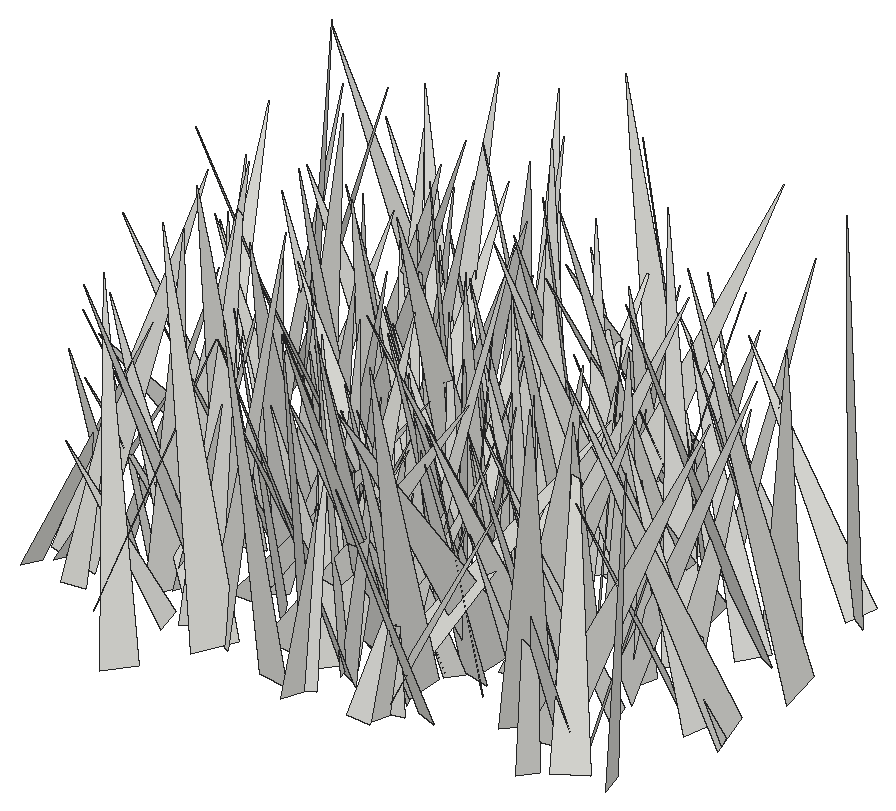
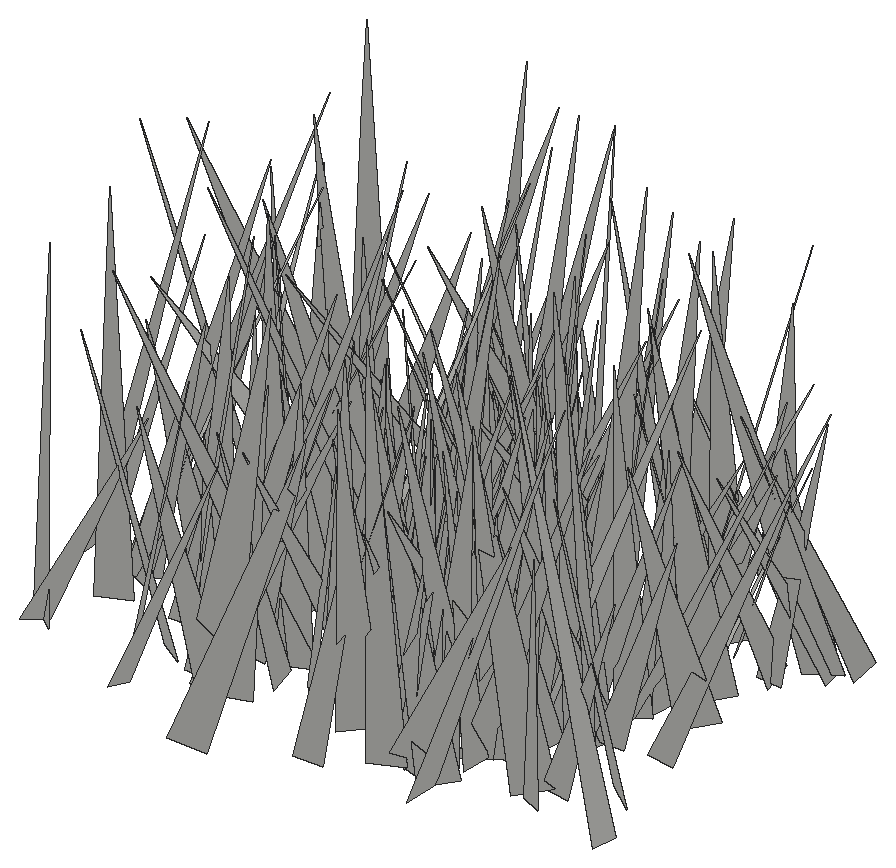
# SketchUp Ruby script. Lengths in inches.
U = 1.inch
M = Sketchup.active_model
def pt(a) = Geom::Point3d.new(a.map { |v| v * U })
def face(e, loops, mat)
  f = e.add_face(loops[0].map { |a| pt(a) })
  loops[1..].each { |l| e.add_face(l.map { |a| pt(a) }).erase! }
  f.material = f.back_material = mat if mat
  f
end
# faces: each face lists its corners as indices into pts; further lists are holes
def faces(e, pts, list, mat = nil) = list.each { |f| face(e, (f[0].is_a?(Array) ? f : [f]).map { |l| l.map { |i| pts[i] } }, mat) }
# xy, xz, yz: faces in a plane at the given z, y or x. An outline is a flat list of corners, or four numbers for a rectangle; further outlines are holes
def ring(l) = l.size == 4 ? [[l[0], l[1]], [l[2], l[1]], [l[2], l[3]], [l[0], l[3]]] : l.each_slice(2).to_a
def flat(e, list, mat, &to3) = list.each { |f| face(e, (f[0].is_a?(Array) ? f : [f]).map { |l| ring(l).map { |u, v| to3.(u, v) } }, mat) }
def xy(e, z, list, mat = nil) = flat(e, list, mat) { |x, y| [x, y, z] }
def xz(e, y, list, mat = nil) = flat(e, list, mat) { |x, z| [x, y, z] }
def yz(e, x, list, mat = nil) = flat(e, list, mat) { |y, z| [x, y, z] }
def lines(e, pts, list) = list.each { |a, b| e.add_line(pt(pts[a]), pt(pts[b])) }
# prism: a flat outline (further loops are holes) pulled along v
def prism(e, loops, v, mat = nil)
  f = face(e, loops, mat); d = Geom::Vector3d.new(v.map { |x| x * U })
  f.pushpull(f.normal.samedirection?(d) ? d.length : -d.length)
end
def box(e, o, s, mat = nil) = prism(e, [[o, [o[0] + s[0], o[1], o[2]], [o[0] + s[0], o[1] + s[1], o[2]], [o[0], o[1] + s[1], o[2]]]], [0, 0, s[2]], mat)
def at(x, y, z, deg = 0) = Geom::Transformation.translation(pt([x, y, z])) * Geom::Transformation.rotation(ORIGIN, Z_AXIS, deg.degrees)
def axes(o, x, y, z) = Geom::Transformation.new([*x, 0, *y, 0, *z, 0, *pt(o).to_a, 1])
def part(name) = M.definitions.add(name)
# library, detail: a bought-in or finely detailed component or shape, given as its bounding box
def library(name, o, s) = part(name).tap { |d| box(d.entities, o, s) }
def detail(e, o, s) = box(e.add_group.entities, o, s)
def put(e, d, t, mat = nil) = e.add_instance(d, t).tap { |i| i.material = mat if mat }
def group(e, t, mat = nil) = e.add_group.tap { |g| g.transformation = t; g.material = mat if mat }.entities
root = M.entities
c1 = part("fur_instance\#9")
p = [[0.8125,0,1.79],[0.67,-0.02,1.48],[0,-0.11,0],[0,0.11,0]]
faces(c1.entities,p,[[0,1,2,3]])
put(root,c1,axes([95.03,323.03,-27.1],[-6.05277,2.56522,0.71834],[2.46544,6.06973,-0.90131],[1.00895,0.55714,6.51184]))
put(root,c1,axes([100.52,325.12,-27.1],[3.76138,-1.24538,0.93866],[-1.27843,-3.86595,-0.00634],[-0.89313,0.28885,3.96218]))
put(root,c1,axes([94.32,326.4375,-27.1],[-3.93279,-0.23592,0.50656],[-0.05149,3.7386,1.34138],[0.55643,-1.32147,3.70448]))
put(root,c1,axes([99.45,325.49,-27.1],[1.25077,5.74635,3.18749],[6.40163,-1.79789,0.7292],[-1.48314,-2.91412,5.83551]))
put(root,c1,axes([99.67,326.98,-27.1],[6.5233,2.37968,3.04495],[3.30026,-6.53866,-1.96019],[-2.01069,-3.01183,6.66138]))
put(root,c1,axes([103.65,327.73,-27.1],[7.48346,-2.4752,1.75576],[-1.96533,-7.51292,-2.21472],[-2.31232,-1.62508,7.56464]))
put(root,c1,axes([104.87,326.64,-27.1],[-1.89303,-4.40404,0.51291],[-4.43222,1.86471,-0.34716],[-0.11875,0.60786,4.78107]))
put(root,c1,axes([103.4,327.9,-27.1],[-5.97447,-2.65496,2.2585],[-2.10106,6.3191,1.8704],[2.78122,-0.92951,6.26456]))
put(root,c1,axes([107.73,328.23,-27.1],[5.80631,-5.6916,0.53269],[-5.68589,-5.82856,-0.29992],[-0.59055,0.15799,8.12513]))
put(root,c1,axes([103.21,325.18,-27.1],[-0.85161,3.55792,0.87868],[3.50079,1.05663,-0.88551],[1.08413,-0.61714,3.54963]))
put(root,c1,axes([103.73,325.76,-27.1],[3.9323,-0.29865,1.47953],[-0.48436,-4.16008,0.44758],[-1.42954,0.58799,3.91814]))
put(root,c1,axes([96.6,326,-27.1],[5.34271,-3.44394,4.19103],[-3.85612,-6.54857,-0.46545],[-3.8152,1.796,6.33945]))
put(root,c1,axes([100.63,325.57,-27.1],[-2.63101,2.88231,1.12737],[2.88894,2.81797,-0.46255],[1.11028,-0.50218,3.87505]))
put(root,c1,axes([101.61,329.17,-27.1],[-1.56855,-7.63886,0.47282],[-7.63369,1.59619,0.46371],[0.55001,0.36889,7.78444]))
put(root,c1,axes([101.04,329.05,-27.1],[-1.24529,-7.71146,0.7872],[-7.61167,1.36728,1.35282],[1.46589,0.54863,7.69333]))
put(root,c1,axes([103.93,326.13,-27.1],[-0.42673,3.51272,1.26133],[3.73148,0.37463,0.21911],[-0.0791,-1.27778,3.53176]))
put(root,c1,axes([93.95,328.97,-27.1],[-5.87667,-3.9224,1.1719],[-3.54254,5.90008,1.98324],[2.05159,-1.04767,6.78139]))
put(root,c1,axes([104.39,331.31,-27.1],[6.48177,-5.01878,0.45242],[-4.24735,-5.8379,-3.90962],[-2.71162,-2.85253,7.2053]))
put(root,c1,axes([90.46,326.36,-27.1],[1.50954,-3.07856,1.78204],[-3.55315,-1.39659,0.59714],[-0.16832,1.87187,3.37633]))
put(root,c1,axes([103.32,326.4,-27.1],[4.26257,2.91433,0.00484],[2.86478,-4.18851,-0.95515],[0.53516,-0.79116,5.0745]))
put(root,c1,axes([101.18,327.18,-27.1],[-4.07281,-4.5818,0.7427],[-4.55178,3.7491,-1.83244],[-0.90871,1.75604,5.85003]))
put(root,c1,axes([110.46,327.26,-27.1],[-2.82559,-5.19892,1.36333],[-5.31081,2.46391,-1.61114],[-0.82624,1.9421,5.69358]))
put(root,c1,axes([101.12,327.32,-27.1],[-2.2184,-4.85625,2.50772],[-5.03427,2.86928,1.10295],[2.1279,1.72546,5.22379]))
put(root,c1,axes([91.81,325.9,-27.1],[4.67763,2.46387,0.32375],[2.42875,-4.67875,0.51598],[-0.52599,0.30722,5.26162]))
put(root,c1,axes([96.28,326.54,-27.1],[3.51282,6.48869,2.15536],[6.79895,-3.57131,-0.32959],[-0.72316,-2.057,7.37118]))
put(root,c1,axes([101.98,329.83,-27.1],[0.91658,-6.09487,0.23316],[-5.96683,-0.94489,-1.24341],[-1.26442,0.04079,6.03668]))
put(root,c1,axes([112.29,326.99,-27.1],[-4.83531,-1.63891,2.39644],[-2.01972,5.24312,-0.48946],[2.08559,1.27782,5.08199]))
put(root,c1,axes([93.04,327.95,-27.1],[-5.61419,2.77509,3.47904],[3.15086,6.4338,-0.04739],[3.14276,-1.49299,6.26243]))
put(root,c1,axes([94.93,328.77,-27.1],[-3.76268,-4.24685,0.11424],[-4.17448,3.66755,-1.15295],[-0.78896,0.84846,5.55555]))
put(root,c1,axes([88.44,326.7,-27.1],[5.14686,-0.10254,0.48257],[-0.21946,-5.00543,1.27711],[-0.44184,1.29176,4.98695]))
put(root,c1,axes([90.48,329.14,-27.1],[-0.08561,-4.51883,0.61864],[-4.55746,0.06047,-0.18896],[-0.17898,0.62161,4.51569]))
put(root,c1,axes([100.42,327.49,-27.1],[-4.38445,3.57185,1.79964],[3.76738,4.58485,0.07863],[1.34299,-1.20052,5.65467]))
put(root,c1,axes([109.75,325.8,-27.1],[-6.16922,0.32467,1.04524],[-0.06119,5.87189,-2.18505],[1.09279,2.16166,5.77844]))
put(root,c1,axes([100.8125,327.64,-27.1],[-6.07164,-2.28107,2.04855],[-2.55827,6.27412,-0.5961],[1.68971,1.3026,6.45854]))
put(root,c1,axes([98.98,329.66,-27.1],[-1.13114,-4.608,0.05517],[-4.59723,1.12439,-0.34274],[-0.31976,0.13515,4.73241]))
put(root,c1,axes([98.36,327.89,-27.1],[4.34126,2.62004,0.01209],[2.52851,-4.18338,-1.34808],[0.68659,-1.1602,4.88813]))
put(root,c1,axes([98.34,327.34,-27.1],[4.70359,-4.43483,0.77561],[-4.1988,-3.91632,3.07011],[1.62462,2.71804,5.6891]))
put(root,c1,axes([110.84,326.64,-27.1],[-3.10471,5.12305,0.88051],[5.18598,3.12286,0.11631],[0.35573,-0.81381,5.98927]))
put(root,c1,axes([97.03,329.07,-27.1],[-4.89402,-3.33819,1.83703],[-3.30827,5.20635,0.64726],[1.89038,0.46913,5.88863]))
put(root,c1,axes([108.12,330.05,-27.1],[-3.94207,-4.94022,1.13908],[-4.81769,4.09962,1.10733],[1.57897,0.1748,6.2225]))
put(root,c1,axes([93.34,328.53,-27.1],[3.78435,-1.32179,0.68035],[-1.35222,-3.83372,0.07338],[-0.61764,0.29457,4.00787]))
put(root,c1,axes([100.32,327.71,-27.1],[-1.02594,6.32348,2.52203],[6.58274,1.57191,-1.26344],[1.73626,-2.22313,6.28034]))
put(root,c1,axes([99.11,329.31,-27.1],[1.24719,-3.91493,0.4967],[-3.8954,-1.13791,0.81231],[0.63182,0.71228,4.02769]))
put(root,c1,axes([100.35,329.27,-27.1],[-1.33091,-4.34516,1.37723],[-4.35803,1.6335,0.94222],[1.33595,0.99989,4.44566]))
put(root,c1,axes([93.37,328.6,-27.1],[0.69074,-4.72184,2.34998],[-4.89788,-1.45354,-1.48096],[-1.95676,1.97148,4.53648]))
put(root,c1,axes([89.04,327.5625,-27.1],[4.0967,-0.1052,0.02727],[-0.10864,-3.93802,1.12914],[0.00278,1.12946,3.93942]))
put(root,c1,axes([94.33,328.06,-27.1],[-2.33068,3.85921,0.35584],[3.66264,2.05758,1.6744],[-1.26695,-1.15111,4.18592]))
put(root,c1,axes([89.42,327.66,-27.1],[0.24663,7.62872,2.41582],[7.70784,0.42293,-2.12242],[2.15005,-2.39126,7.33168]))
put(root,c1,axes([104.46,329.69,-27.1],[-2.38494,-6.16406,1.52656],[-6.35023,2.30898,-0.59758],[-0.0234,1.63919,6.58229]))
put(root,c1,axes([108.95,327.74,-27.1],[5.79439,-3.93356,1.43708],[-4.17619,-5.2444,2.48372],[0.31237,2.85246,6.54821]))
put(root,c1,axes([92.67,328,-27.1],[-3.84784,-1.19504,0.32807],[-1.23606,3.62421,-1.29571],[-0.08892,1.33363,3.81512]))
put(root,c1,axes([106.33,329.93,-27.1],[-3.36385,-0.86607,1.07357],[-0.51946,3.41676,1.12873],[1.27781,-0.89095,3.28504]))
put(root,c1,axes([103.16,329.6,-27.1],[-3.34237,-3.67886,0.49489],[-3.71061,3.29315,-0.58039],[-0.10119,0.75599,4.93646]))
put(root,c1,axes([91.96,330.39,-27.1],[-3.17916,-2.57933,0.00353],[-2.53731,3.12837,0.73174],[0.46373,-0.56605,4.02798]))
put(root,c1,axes([105.08,329.23,-27.1],[-3.3946,-3.12525,1.18102],[-3.29173,3.41661,-0.4203],[0.5714,1.11577,4.59499]))
put(root,c1,axes([105.97,331.33,-27.1],[2.24091,-5.47361,0.67385],[-5.23088,-2.33999,-1.61199],[-1.7471,-0.01469,5.69066]))
put(root,c1,axes([98.25,328.7,-27.1],[4.49912,0.07902,0.02983],[0.07502,-4.46879,0.52292],[-0.03881,0.52233,4.46932]))
put(root,c1,axes([97.99,330.15,-27.1],[1.8485,-3.49978,1.33816],[-3.45042,-2.17169,-0.91344],[-1.46071,0.70098,3.8511]))
put(root,c1,axes([110.15,332.93,-27.1],[-3.50557,-5.51536,0.11612],[-4.95597,3.20905,2.80393],[2.42302,-1.41579,5.90306]))
put(root,c1,axes([106.26,330.34,-27.1],[2.2039,-6.87435,1.74953],[-7.02125,-1.85328,1.56272],[1.00974,2.1174,7.04782]))
put(root,c1,axes([103.87,329.39,-27.1],[-0.77186,4.35622,1.72795],[4.2436,-0.09339,2.13104],[-1.98854,-1.8902,3.87699]))
put(root,c1,axes([113.22,331.94,-27.1],[-7.42684,-1.75978,1.28146],[-1.36577,7.3143,2.12899],[1.69519,-1.81689,7.32954]))
put(root,c1,axes([109.69,330.6,-27.1],[-5.35424,-1.86738,0.02315],[-1.86377,5.3475,0.29345],[0.11847,-0.26947,5.66294]))
put(root,c1,axes([95.07,332.36,-27.1],[7.37439,-3.31849,1.28024],[-2.90244,-7.31769,-2.24953],[-2.05603,-1.57231,7.76747]))
put(root,c1,axes([102.41,327.58,-27.1],[0.90469,6.24799,0.05202],[5.52251,-0.775,-2.9597],[2.92267,-0.46962,5.57638]))
put(root,c1,axes([95.3,326.83,-27.1],[-7.34828,2.49323,1.09592],[2.03506,7.1224,-2.5582],[1.80991,2.11416,7.32591]))
put(root,c1,axes([97.38,331.02,-27.1],[2.10827,-4.41232,0.88185],[-4.4927,-2.11805,0.1432],[-0.24874,0.85808,4.88803]))
put(root,c1,axes([101.06,329.68,-27.1],[1.63148,3.88333,0.8996],[3.80186,-1.22375,-1.61232],[1.19808,-1.40479,3.89132]))
put(root,c1,axes([107.17,331.95,-27.1],[1.92624,-6.27783,0.49509],[-6.26935,-1.863,0.76884],[0.59288,0.69623,6.52153]))
put(root,c1,axes([101.15,332.76,-27.1],[5.45875,-2.61976,0.1584],[-2.41646,-5.15945,-2.05595],[-1.02417,-1.78972,5.6951]))
put(root,c1,axes([104.25,333.1,-27.1],[-5.79035,-4.99721,0.36352],[-4.82955,5.71454,1.62848],[1.33407,-1.00217,7.47317]))
put(root,c1,axes([93.13,331.75,-27.1],[2.46891,-7.20313,1.70316],[-7.36136,-2.57683,-0.22704],[-0.77207,1.53499,7.61111]))
put(root,c1,axes([92.8,329.42,-27.1],[3.62084,3.81527,1.03017],[3.87963,-3.69771,0.05854],[-0.75237,-0.70613,5.25959]))
put(root,c1,axes([105.57,330.55,-27.1],[3.73995,-4.97965,1.07609],[-4.97131,-3.27521,2.12161],[1.114,2.10195,5.85517]))
put(root,c1,axes([90.45,328.75,-27.1],[4.99403,0.89918,1.35491],[0.3935,-4.91429,1.81096],[-1.5778,1.62046,4.74018]))
put(root,c1,axes([95.3125,329.14,-27.1],[4.61387,-2.10989,0.31356],[-1.93342,-3.82099,2.73855],[0.90102,2.60502,4.2708]))
put(root,c1,axes([96.03,330.08,-27.1],[3.36091,-1.13304,0.9234],[-1.35023,-3.29337,0.87337],[-0.55977,1.1411,3.43755]))
put(root,c1,axes([94.78,331.9,-27.1],[-2.52034,-4.28654,0.32351],[-4.12689,2.30776,-1.57296],[-1.20326,1.06349,4.71724]))
put(root,c1,axes([113.24,331.73,-27.1],[-6.30191,-3.29477,0.26908],[-3.30318,6.25333,-0.79169],[-0.13009,0.82599,7.06702]))
put(root,c1,axes([98.65,331.99,-27.1],[-4.19066,-2.50752,1.09961],[-2.47633,4.32875,0.43379],[1.16817,0.18082,4.86427]))
put(root,c1,axes([112.28,331.59,-27.1],[-4.9541,1.83691,1.27432],[2.05779,4.95762,0.85363],[0.87385,-1.26054,5.21428]))
put(root,c1,axes([102.53,327.9,-27.1],[3.62911,6.60842,0.2466],[6.35712,-3.56375,1.94657],[-1.82181,0.72867,7.28371]))
put(root,c1,axes([91.14,331.22,-27.1],[5.12672,-4.5376,2.59386],[-5.0883,-5.16347,1.02416],[-1.19461,2.5199,6.76936]))
put(root,c1,axes([98.95,333.11,-27.1],[-3.68425,-5.36529,0.32526],[-5.32374,3.58793,-1.11818],[-0.74155,0.8979,6.41168]))
put(root,c1,axes([103.25,332.38,-27.1],[-1.22069,-3.41408,1.05948],[-3.55821,1.26785,-0.01408],[0.34288,1.00256,3.62571]))
put(root,c1,axes([99.66,332.62,-27.1],[-3.20699,2.34244,2.63387],[2.95903,3.72406,0.29089],[1.91533,-1.83124,3.96071]))
put(root,c1,axes([108.55,332.3,-27.1],[4.54413,5.8348,1.67226],[5.93472,-3.83302,-2.75273],[1.27295,-2.95864,6.86415]))
put(root,c1,axes([103.3125,332.32,-27.1],[-0.92871,-3.83483,1.6083],[-4.04735,1.2119,0.55253],[0.95473,1.40727,3.90681]))
put(root,c1,axes([89.95,335.42,-27.1],[4.40481,-2.70951,0.82389],[-1.71706,-3.76665,-3.20728],[-2.2521,-2.42766,4.05674]))
put(root,c1,axes([96.76,332.57,-27.1],[0.02782,-4.7345,1.86898],[-5.06027,0.17616,0.52158],[0.54982,1.86087,4.70577]))
put(root,c1,axes([108.96,332.86,-27.1],[3.6892,-1.49713,1.29137],[-1.47127,-3.90506,-0.32413],[-1.32076,0.16824,3.96818]))
put(root,c1,axes([92.43,333.74,-27.1],[2.19919,-5.46865,1.19281],[-5.58851,-2.07385,0.79564],[0.31218,1.39943,5.84033]))
put(root,c1,axes([92.4,333.75,-27.1],[-5.87087,-0.65311,0.1721],[-0.62527,5.82501,0.77566],[0.25536,-0.75237,5.85594]))
put(root,c1,axes([104.39,331.61,-27.1],[3.12045,6.97557,0.92804],[6.87353,-2.80376,-2.03727],[1.5081,-1.6545,7.36514]))
put(root,c1,axes([110.32,328.2,-27.1],[5.94606,5.36025,0.59468],[4.2161,-5.17199,4.4628],[-3.36309,2.9933,6.64615]))
put(root,c1,axes([92,332.57,-27.1],[-5.13165,1.21269,1.54361],[1.09048,5.35359,-0.58061],[1.63224,0.23592,5.24093]))
put(root,c1,axes([106.85,334.33,-27.1],[2.3512,-5.85332,1.44977],[-6.03015,-2.28819,0.5412],[-0.02311,1.54732,6.28463]))
put(root,c1,axes([100.87,333.83,-27.1],[4.61711,2.95667,1.94744],[3.35791,-4.67134,-0.86895],[-1.12198,-1.8135,5.41336]))
put(root,c1,axes([99.21,332.71,-27.1],[-3.06534,4.86368,0.18481],[4.51167,2.75744,2.26433],[-1.82603,-1.35165,5.28436]))
put(root,c1,axes([101.11,334.03,-27.1],[4.30698,0.82715,0.77594],[0.97071,-4.26434,-0.84231],[-0.5865,-0.98365,4.30404]))
put(root,c1,axes([100.98,333.84,-27.1],[-2.4507,-4.58404,1.24543],[-4.71435,2.17524,-1.27033],[-0.58261,1.68089,5.0404]))
put(root,c1,axes([106.03,334.03,-27.1],[4.89735,3.35239,2.18214],[3.80193,-4.97328,-0.89225],[-1.24321,-2.00306,5.86741]))
put(root,c1,axes([104.77,331.99,-27.1],[1.00631,5.78428,1.17144],[5.41169,-1.37849,2.15781],[-2.35451,-0.6962,5.46025]))
put(root,c1,axes([94.97,335.56,-27.1],[-4.99858,-6.00178,0.67378],[-6.03784,4.94565,-0.739],[-0.1407,0.9901,7.77567]))
put(root,c1,axes([106.64,336.25,-27.1],[-7.7703,-1.5883,1.42664],[-1.2052,7.70803,2.01725],[1.76224,-1.7318,7.67014]))
put(root,c1,axes([93.95,334.08,-27.1],[-5.48132,1.03762,0.48302],[1.07413,5.47965,0.41785],[0.39525,-0.50168,5.563]))
put(root,c1,axes([94.95,334.65,-27.1],[5.5976,-0.64404,1.05715],[-0.59203,-5.69245,-0.3332],[-1.08713,-0.21617,5.62467]))
put(root,c1,axes([93.49,335.75,-27.1],[0.81031,-5.69395,0.84212],[-5.55553,-0.55126,1.61834],[1.50543,1.03047,5.51893]))
put(root,c1,axes([110.77,336.59,-27.1],[-3.23676,-6.95107,0.75182],[-6.9834,3.25434,0.02332],[0.33861,0.67166,7.66769]))
put(root,c1,axes([93.72,335.43,-27.1],[-0.85908,-3.57953,0.71794],[-3.54097,0.99653,0.73143],[0.88884,0.51028,3.60778]))
put(root,c1,axes([99.27,334.42,-27.1],[-4.79619,2.23097,0.90337],[2.34699,4.78153,0.65218],[0.53379,-0.97799,5.24932]))
put(root,c1,axes([113.23,335.6,-27.1],[-7.82049,-1.65264,1.82204],[-1.48703,8.01344,0.88582],[1.95953,-0.51451,7.94397]))
put(root,c1,axes([94.43,336.13,-27.1],[6.50516,0.09741,3.11354],[0.81371,-7.01185,-1.48071],[-3.00691,-1.68675,6.33514]))
put(root,c1,axes([104.8125,334.34,-27.1],[3.28542,-2.52777,1.83261],[-2.97263,-3.34603,0.71392],[-0.95477,1.71946,4.08337]))
put(root,c1,axes([93.3125,335.03,-27.1],[6.93717,-2.75986,2.51351],[-2.97128,-7.29338,0.19237],[-2.25967,1.11744,7.46352]))
put(root,c1,axes([102.1,335.58,-27.1],[1.8151,-3.86013,1.55176],[-3.9232,-2.15155,-0.76319],[-1.38458,1.03602,4.19675]))
put(root,c1,axes([100.08,333.6,-27.1],[3.50829,2.33455,0.59392],[2.17247,-3.51961,1.00185],[-1.04078,0.52272,4.09323]))
put(root,c1,axes([100.59,333.42,-27.1],[-4.5545,1.12209,0.15618],[1.0267,4.36161,-1.39615],[0.47894,1.3207,4.4781]))
put(root,c1,axes([97.65,338.08,-27.1],[7.10031,-2.91459,1.55919],[-2.29482,-7.00551,-2.64516],[-2.37902,-1.94118,7.20502]))
put(root,c1,axes([100.1875,334.35,-27.1],[-4.76219,-1.42096,1.84075],[-1.91994,4.76946,-1.2853],[1.31199,1.82182,4.80058]))
put(root,c1,axes([112.125,336.68,-27.1],[-3.86878,-4.9807,0.99535],[-5.05831,3.89149,-0.18804],[0.45997,0.9025,6.30392]))
put(root,c1,axes([90.42,332.86,-27.1],[-4.33285,5.33033,0.39838],[5.19442,4.31986,-1.30443],[1.26061,0.52067,6.74422]))
put(root,c1,axes([108.9,335.21,-27.1],[4.04203,-2.33275,1.48439],[-2.65208,-4.01454,0.91276],[-0.78205,1.55722,4.57675]))
put(root,c1,axes([99.34,335.74,-27.1],[-3.99444,1.28958,0.25526],[1.31279,3.95594,0.55757],[0.06915,-0.60932,4.16025]))
put(root,c1,axes([91.93,335.63,-27.1],[-2.38269,3.95567,1.05235],[4.03891,2.07425,1.34786],[-0.66484,-1.57548,4.41677]))
put(root,c1,axes([107.99,337.96,-27.1],[3.38324,-1.277,0.34003],[-0.90165,-2.91389,-1.97203],[-0.96612,-1.75247,3.03119]))
put(root,c1,axes([98.84,335.94,-27.1],[-5.61783,-2.93903,2.21928],[-3.25584,5.85535,-0.48739],[1.72124,1.48327,6.32142]))
put(root,c1,axes([98.36,337.33,-27.1],[1.13187,-5.42392,1.09616],[-5.52646,-1.05128,0.50466],[0.2806,1.17367,5.51773]))
put(root,c1,axes([98.62,335.11,-27.1],[-5.41908,-0.82486,1.13145],[-1.12996,5.24719,-1.58656],[0.82691,1.76453,5.24687]))
put(root,c1,axes([106.2,336.35,-27.1],[-3.46887,0.5768,0.94943],[0.60796,3.5911,0.03958],[0.92978,-0.19616,3.51628]))
put(root,c1,axes([110.52,338.06,-27.1],[1.17808,-6.7396,1.1437],[-6.76699,-0.98532,1.16408],[0.96855,1.31342,6.74203]))
put(root,c1,axes([110.67,336.37,-27.1],[-3.89894,3.87426,1.21258],[4.05705,3.77806,0.97396],[0.14352,-1.54866,5.40953]))
put(root,c1,axes([109.18,334.59,-27.1],[-7.08431,2.74004,0.68893],[2.60293,7.0529,-1.28499],[1.09872,0.95845,7.48626]))
put(root,c1,axes([96.21,336.18,-27.1],[6.43486,-0.85229,1.84553],[-1.08084,-6.62327,0.70985],[-1.72168,0.97247,6.45212]))
put(root,c1,axes([97.52,336.16,-27.1],[-3.69275,-0.52533,1.17947],[-0.76187,3.77166,-0.70545],[1.04243,0.89562,3.66261]))
put(root,c1,axes([93.67,338.36,-27.1],[3.36896,-5.0045,1.18358],[-5.04079,-3.49374,-0.42432],[-1.01802,0.73793,6.01788]))
put(root,c1,axes([92.1,335.65,-27.1],[4.14579,-2.60609,2.17076],[-3.31381,-3.84297,1.71517],[-0.72292,2.67047,4.58667]))
put(root,c1,axes([95.92,337.82,-27.1],[-2.42816,-5.42807,1.43938],[-5.61543,2.33238,-0.67728],[-0.05217,1.5899,5.90772]))
put(root,c1,axes([92.36,335.8,-27.1],[-7.10447,-2.39928,3.44832],[-3.25719,7.42464,-1.54476],[2.65295,2.69055,7.33783]))
put(root,c1,axes([96.46,336.18,-27.1],[-4.11869,2.39634,0.55767],[2.352,4.15398,-0.47915],[0.72219,0.13795,4.74094]))
put(root,c1,axes([93.34,337.16,-27.1],[7.44021,-1.05618,0.97458],[-1.13327,-7.472,0.55406],[-0.88376,0.68976,7.49435]))
put(root,c1,axes([105.98,338.32,-27.1],[-1.13695,-6.80591,1.9758],[-6.92615,0.64332,-1.76957],[-1.50086,2.18691,6.66945]))
put(root,c1,axes([98,336.64,-27.1],[-3.61656,3.24074,0.55892],[3.26072,3.64166,-0.01623],[0.42715,-0.36083,4.85609]))
put(root,c1,axes([94.75,339.04,-27.1],[-5.48359,2.23586,1.70204],[2.68404,5.27249,1.72124],[0.83185,-2.27324,5.66623]))
put(root,c1,axes([105.73,339.01,-27.1],[2.79472,-2.37927,0.19168],[-2.37504,-2.80125,-0.14262],[-0.23842,0.01542,3.66757]))
put(root,c1,axes([98.94,339.12,-27.1],[-4.40075,-1.21691,1.44212],[-0.98766,4.60363,0.87078],[1.60783,-0.50284,4.4821]))
put(root,c1,axes([95.34,336.95,-27.1],[-1.64071,6.20292,1.41522],[6.35653,1.66047,0.09149],[0.27128,-1.39198,6.41559]))
put(root,c1,axes([91.86,339.59,-27.1],[3.71453,-6.09838,0.78607],[-6.05056,-3.46164,1.73599],[1.09493,1.55972,6.92635]))
put(root,c1,axes([101.55,339.1,-27.1],[-4.35453,-4.53446,2.05004],[-4.74623,4.60317,0.10013],[1.49574,1.4055,6.28595]))
put(root,c1,axes([103.41,337.67,-27.1],[-5.08391,3.17186,1.29588],[3.17676,5.23223,-0.34381],[1.28383,-0.38638,5.98237]))
put(root,c1,axes([102.27,337.33,-27.1],[-6.74391,-2.32387,0.77011],[-2.44649,6.31426,-2.37034],[-0.09,2.49068,6.72772]))
put(root,c1,axes([106.95,338.67,-27.1],[-6.4254,-4.61842,2.37343],[-5.01235,6.50279,-0.91585],[1.35622,2.15235,7.85982]))
put(root,c1,axes([96.59,335.48,-27.1],[-4.56686,4.07542,0.09193],[3.68922,4.19072,-2.51023],[1.73411,1.8173,5.58247]))
put(root,c1,axes([98.3,337.23,-27.1],[-2.89622,3.26829,0.45856],[3.08153,2.89643,-1.18106],[1.18158,0.4572,4.20415]))
put(root,c1,axes([101.58,336.57,-27.1],[-1.51981,5.35977,0.02073],[5.22969,1.48762,-1.21441],[1.17387,0.31183,5.43711]))
put(root,c1,axes([100.94,338.16,-27.1],[-0.82841,6.75025,1.93378],[7.00258,0.65031,0.72978],[-0.51887,-2.00072,6.76162]))
put(root,c1,axes([94.92,340.26,-27.1],[4.55576,-0.64185,1.19418],[-0.37344,-4.61891,-1.05794],[-1.3033,-0.92017,4.47746]))
put(root,c1,axes([104.77,338.29,-27.1],[-1.73609,5.26171,0.91511],[5.1615,1.40586,1.70864],[-1.37182,-1.3693,5.27069]))
put(root,c1,axes([94.49,339.36,-27.1],[5.43956,-0.0104,1.6458],[0.01524,-5.68242,-0.08629],[-1.64576,-0.087,5.43889]))
put(root,c1,axes([104.83,340.98,-27.1],[-2.5051,-3.46967,0.23869],[-3.39401,2.50314,0.76559],[0.75915,-0.25846,4.21047]))
put(root,c1,axes([104.36,341.24,-27.1],[-1.56968,-5.60909,0.11931],[-5.50885,1.51747,-1.1357],[-1.06238,0.41882,5.71278]))
put(root,c1,axes([87.98,340.79,-27.1],[8.03575,1.73258,0.69022],[1.85682,-7.7181,-2.24381],[-0.17451,-2.34107,7.90825]))
put(root,c1,axes([91.3,339.21,-27.1],[-1.35537,3.98703,1.26023],[4.07237,0.95801,1.34893],[-0.94888,-1.58348,3.98921]))
put(root,c1,axes([89.47,338.125,-27.1],[3.26782,5.25044,1.3347],[5.28581,-3.43164,0.55786],[-1.18691,-0.82697,6.1591]))
put(root,c1,axes([96.74,338.05,-27.1],[-5.17368,4.83178,0.63052],[4.85594,5.1888,0.08232],[0.40437,-0.49072,7.07858]))
put(root,c1,axes([102.85,337.86,-27.1],[1.48421,7.77893,1.22221],[7.56365,-1.06243,-2.42301],[2.19017,-1.60247,7.53948]))
put(root,c1,axes([94.6,341.11,-27.1],[3.61715,-5.66391,0.01487],[-5.50634,-3.51236,1.58351],[1.3268,0.86448,6.53117]))
put(root,c1,axes([103.3,340.8,-27.1],[2.16413,-4.87719,1.14426],[-4.95965,-2.26151,-0.2591],[-0.70577,0.93721,5.32947]))
put(root,c1,axes([102.84,338.91,-27.1],[4.75143,0.92242,1.33841],[0.70934,-4.89704,0.85681],[-1.46255,0.62163,4.7637]))
put(root,c1,axes([96.75,341.17,-27.1],[1.17018,-6.95871,1.51726],[-7.0392,-0.89595,1.31981],[1.08411,1.69372,6.93189]))
put(root,c1,axes([99.89,337.26,-27.1],[-6.30964,2.41528,1.06239],[1.96226,6.1361,-2.29599],[1.76402,1.81341,6.35402]))
put(root,c1,axes([96.51,340.75,-27.1],[-2.7828,-3.97435,1.2381],[-4.07565,2.90431,0.16237],[0.84701,0.91751,4.84903]))
put(root,c1,axes([95.79,338.21,-27.1],[0.08321,7.29137,1.2347],[7.39423,-0.10178,0.10277],[-0.11831,-1.23331,7.29112]))
put(root,c1,axes([97.23,340.3125,-27.1],[-3.6032,0.74818,1.09352],[0.87855,3.72087,0.34907],[0.99182,-0.57787,3.66346]))
put(root,c1,axes([91.48,340.26,-27.1],[-1.7362,-3.80786,1.79903],[-4.13168,1.91701,0.07019],[0.81577,1.60498,4.18441]))
put(root,c1,axes([98.87,342.56,-27.1],[-0.42981,-6.03201,0.26249],[-6.01913,0.44871,0.45551],[0.47339,0.22867,6.03012]))
put(root,c1,axes([111.65,340.73,-27.1],[-4.58774,2.19144,0.09862],[2.15217,4.45217,1.18567],[-0.42461,-1.11142,4.94408]))
put(root,c1,axes([106.79,339.75,-27.1],[3.4607,5.10853,1.2476],[5.25066,-3.43918,-0.48234],[-0.29016,-1.30574,6.15149]))
put(root,c1,axes([107.4375,341.08,-27.1],[-4.91949,-2.25789,1.34677],[-2.33985,5.06309,-0.05864],[1.19873,0.61667,5.41258]))
put(root,c1,axes([111.65,340.42,-27.1],[-3.98091,-5.38333,3.048],[-6.04161,4.16252,-0.53901],[1.33021,2.79489,6.67363]))
put(root,c1,axes([104.03,340.97,-27.1],[3.98681,-3.04122,0.56389],[-3.08769,-3.85909,1.01744],[0.18196,1.14894,4.91004]))
put(root,c1,axes([94.67,341.93,-27.1],[-7.8071,-1.03462,1.04066],[-0.93299,7.84786,0.80297],[1.13267,-0.66693,7.83431]))
put(root,c1,axes([102.57,344.23,-27.1],[3.27442,-5.47757,0.11686],[-5.10679,-3.10069,-2.24625],[-1.98447,-1.05885,5.97327]))
put(root,c1,axes([104.73,340.29,-27.1],[-3.07753,7.46975,2.03134],[7.70521,2.74591,1.57617],[-0.74375,-2.46119,7.92363]))
put(root,c1,axes([98.875,339.84,-27.1],[-4.66477,5.25581,1.41142],[5.28211,4.8201,-0.49149],[1.30953,-0.72026,7.01013]))
put(root,c1,axes([96.17,340.93,-27.1],[-1.67581,5.69721,1.32161],[5.39716,0.9769,2.63242],[-2.25291,-1.89755,5.32325]))
put(root,c1,axes([106.84,342.4,-27.1],[-4.54566,0.43172,0.55069],[0.54174,4.46219,0.97364],[0.44289,-1.02717,4.4611]))
